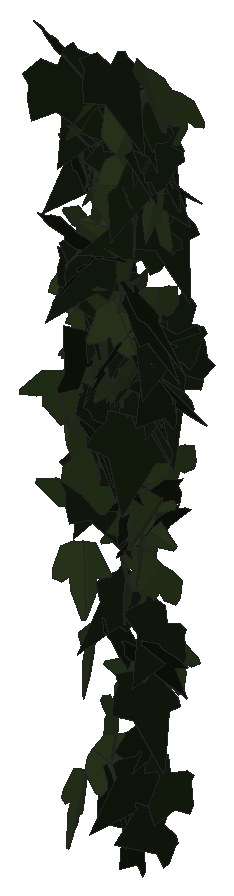
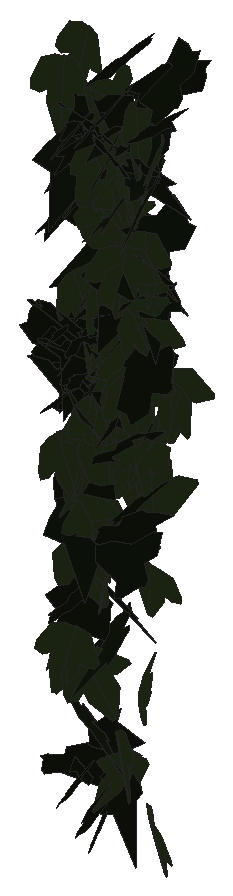
# SketchUp Ruby script. Lengths in inches.
U = 1.inch
M = Sketchup.active_model
def pt(a) = Geom::Point3d.new(a.map { |v| v * U })
def face(e, loops, mat)
  f = e.add_face(loops[0].map { |a| pt(a) })
  loops[1..].each { |l| e.add_face(l.map { |a| pt(a) }).erase! }
  f.material = f.back_material = mat if mat
  f
end
# faces: each face lists its corners as indices into pts; further lists are holes
def faces(e, pts, list, mat = nil) = list.each { |f| face(e, (f[0].is_a?(Array) ? f : [f]).map { |l| l.map { |i| pts[i] } }, mat) }
# xy, xz, yz: faces in a plane at the given z, y or x. An outline is a flat list of corners, or four numbers for a rectangle; further outlines are holes
def ring(l) = l.size == 4 ? [[l[0], l[1]], [l[2], l[1]], [l[2], l[3]], [l[0], l[3]]] : l.each_slice(2).to_a
def flat(e, list, mat, &to3) = list.each { |f| face(e, (f[0].is_a?(Array) ? f : [f]).map { |l| ring(l).map { |u, v| to3.(u, v) } }, mat) }
def xy(e, z, list, mat = nil) = flat(e, list, mat) { |x, y| [x, y, z] }
def xz(e, y, list, mat = nil) = flat(e, list, mat) { |x, z| [x, y, z] }
def yz(e, x, list, mat = nil) = flat(e, list, mat) { |y, z| [x, y, z] }
def lines(e, pts, list) = list.each { |a, b| e.add_line(pt(pts[a]), pt(pts[b])) }
# prism: a flat outline (further loops are holes) pulled along v
def prism(e, loops, v, mat = nil)
  f = face(e, loops, mat); d = Geom::Vector3d.new(v.map { |x| x * U })
  f.pushpull(f.normal.samedirection?(d) ? d.length : -d.length)
end
def box(e, o, s, mat = nil) = prism(e, [[o, [o[0] + s[0], o[1], o[2]], [o[0] + s[0], o[1] + s[1], o[2]], [o[0], o[1] + s[1], o[2]]]], [0, 0, s[2]], mat)
def at(x, y, z, deg = 0) = Geom::Transformation.translation(pt([x, y, z])) * Geom::Transformation.rotation(ORIGIN, Z_AXIS, deg.degrees)
def axes(o, x, y, z) = Geom::Transformation.new([*x, 0, *y, 0, *z, 0, *pt(o).to_a, 1])
def part(name) = M.definitions.add(name)
# library, detail: a bought-in or finely detailed component or shape, given as its bounding box
def library(name, o, s) = part(name).tap { |d| box(d.entities, o, s) }
def detail(e, o, s) = box(e.add_group.entities, o, s)
def put(e, d, t, mat = nil) = e.add_instance(d, t).tap { |i| i.material = mat if mat }
def group(e, t, mat = nil) = e.add_group.tap { |g| g.transformation = t; g.material = mat if mat }.entities
root = M.entities
M.materials.add("efeu1").color = [18, 25, 13]
M.materials.add("efeu2").color = [43, 57, 29]
c1 = part("ivyleaf_10")
p = [[0,0.5,-0.03],[-0.0625,2.02,-0.43],[-0.19,2.01,-0.46],[-0.54,1.05,-0.29],[-0.52,0.625,-0.18],[-0.83,0.76,-0.28],
  [-1.16,0.64,-0.33],[-1.15,0.33,-0.24],[-0.77,-0.39,0.02],[-0.3,-0.51,0.16],[0.04,-0.48,0.23],[-0.02,2.01,-0.4375],
  [-0.06,2.01,-0.43],[0.04,-0.49,0.23],[0.67,-0.49,0.14],[1.38,0.36,-0.2],[1.375,0.51,-0.24],[0.81,0.65,-0.19],
  [0.62,0.59,-0.15],[0.6,1.09,-0.28],[0.5,1.23,-0.31]]
faces(c1.entities,p,[[0,1,2,3,4,5,6,7,8,9,10],[11,12,0,13,14,15,16,17,18,19,20]],"efeu2")
c2 = part("ivyleaf_9")
p = [[1.54,2.16,1.25],[1.36,2.04,1.19],[-0.21,0.99,0.68],[-0.71,1.11,0.82],[-0.85,0.86,0.67],[-0.8,0.17,0.21],
  [-0.9,-0.01,0.1],[-0.67,-0.16,-0.02],[-0.08,-0.08,-0.05],[-0.03,-0.6,-0.4],[0.65,-0.88,-0.66],[0.83,-0.6,-0.49],
  [1.29,-0.42,-0.43],[1.8125,-0.07,-0.26],[1.21,0.44,0.15]]
faces(c2.entities,p,[[0,1,2,3,4,5,6,7,8,9,10,11,12,13,14]],"efeu1")
put(root,c1,axes([551.82,132.52,225.93],[0.90272,0.27085,-0.02157],[-0.0193,-0.01073,-0.94246],[-0.27102,0.90291,-0.00473]))
put(root,c1,axes([551.79,132.23,207.72],[0.74606,-0.58457,0.23749],[0.18704,-0.14635,-0.9478],[0.60261,0.76915,0.00016]))
put(root,c1,axes([551.89,131.1,222.64],[-0.84438,0.29558,-0.21811],[0.19346,-0.10696,-0.8939],[-0.31227,-0.86551,0.03597]))
put(root,c1,axes([552.12,130.91,223.07],[-0.61057,-0.69177,-0.01816],[0.01288,0.01285,-0.92268],[0.69189,-0.6107,0.00115]))
put(root,c2,axes([551.3,131.7,234.54],[0.67517,-0.64526,0.39472],[0.33513,-0.21915,-0.93149],[0.67812,0.75075,0.06735]))
put(root,c1,axes([552.12,132.82,226.29],[-0.06301,-0.82511,0.44369],[0.0616,-0.44737,-0.82322],[0.93481,-0.02613,0.08415]))
put(root,c2,axes([551.42,132.96,224.04],[0.98155,-0.02971,-0.34505],[0.34599,0.12956,0.97308],[0.01517,-1.03233,0.13205]))
put(root,c2,axes([552.12,131.72,231.09],[0.5706,-0.13273,-0.74714],[-0.6309,0.43646,-0.55937],[0.42166,0.83266,0.17411]))
put(root,c1,axes([552.34,132.76,223.61],[-0.46458,-0.79522,0.11666],[-0.01288,-0.12737,-0.91947],[0.80363,-0.46176,0.0527]))
put(root,c2,axes([552.27,133.3125,219],[-0.52467,-0.73699,0.09525],[-0.02342,-0.10014,-0.90384],[0.74275,-0.52376,0.03878]))
put(root,c2,axes([552.59,131.42,226.9375],[-0.1355,0.93298,0.12548],[-0.00562,0.12597,-0.94269],[-0.94137,-0.13505,-0.01243]))
put(root,c1,axes([552.57,131.87,228.29],[-0.89062,0.05393,0.30576],[-0.30524,0.01773,-0.89226],[-0.05676,-0.94148,0.00072]))
put(root,c1,axes([552.375,132.62,223.84],[-0.57631,-0.75007,0.02522],[0.07123,-0.08632,-0.93961],[0.74711,-0.57037,0.10903]))
put(root,c2,axes([551.84,132.36,226.375],[0.32161,-0.89231,0.10139],[0.05079,-0.08945,-0.94834],[0.89662,0.32513,0.01736]))
put(root,c1,axes([552.25,131.57,231.69],[-0.48634,0.81522,0.00802],[0.00541,0.01257,-0.9492],[-0.81524,-0.48624,-0.01108]))
put(root,c1,axes([552.01,132.53,212.6875],[0.10473,-0.36689,0.82699],[0.58913,-0.60416,-0.34264],[0.68662,0.57434,0.16785]))
put(root,c1,axes([552.18,132.22,221.23],[0.4325,0.71572,0.44173],[0.21496,0.38615,-0.83613],[-0.81313,0.48277,0.01391]))
put(root,c1,axes([552.6,131.35,221.3],[0.09304,0.56348,0.72436],[-0.29807,0.70716,-0.51182],[-0.86797,-0.18244,0.2534]))
put(root,c2,axes([552.4,132.27,232.56],[-0.36839,-0.80212,0.38113],[-0.00085,-0.41231,-0.86855],[0.88807,-0.33313,0.15728]))
put(root,c2,axes([552.15,130.82,234.28],[0.13921,-0.73438,-0.69502],[-0.01521,0.69998,-0.74267],[1.01101,0.11165,0.08453]))
put(root,c2,axes([552.93,131.98,231.07],[-0.93048,-0.15791,0.00198],[-0.00094,-0.00629,-0.94377],[0.15792,-0.93046,0.00604]))
put(root,c1,axes([552.6875,132.625,224.95],[-0.48953,-0.7833,0.20194],[0.01391,-0.24416,-0.91333],[0.80879,-0.4699,0.13794]))
put(root,c1,axes([552.75,132.4,227.34],[-0.50526,-0.80101,-0.05026],[0.06353,0.01929,-0.94606],[0.80007,-0.50739,0.04338]))
put(root,c1,axes([552.37,131.6,216.45],[0.91454,-0.01963,0.28681],[0.28667,-0.00966,-0.91474],[0.02162,0.95841,-0.00335]))
put(root,c2,axes([552.6,133.16,221.54],[-0.36059,-0.83056,0.17307],[0.00773,-0.19126,-0.90176],[0.84836,-0.35128,0.08178]))
put(root,c2,axes([551.95,132.71,217.49],[0.58855,-0.42318,0.60133],[0.52116,-0.30329,-0.72352],[0.51872,0.78486,0.04464]))
put(root,c1,axes([552.93,132.49,210.43],[0.54202,-0.50406,-0.50402],[-0.25961,0.45011,-0.72932],[0.66387,0.58756,0.12631]))
put(root,c1,axes([552.75,131.14,218.91],[-0.94233,-0.44249,0.09803],[0.0915,0.03576,1.04103],[-0.44389,0.94674,0.0065]))
put(root,c1,axes([552.87,131.72,232.84],[0.02812,-0.9489,-0.20865],[0.01447,0.20912,-0.9491],[0.97146,0.02435,0.02018]))
put(root,c2,axes([553.125,131.6875,227.49],[-0.94346,-0.08712,-0.10658],[0.1105,-0.0391,-0.94621],[0.08208,-0.94865,0.04879]))
put(root,c2,axes([552.71,131.4,223.55],[0.22376,0.39828,0.90514],[-0.43122,-0.79584,0.45679],[0.88992,-0.48577,-0.00625]))
put(root,c1,axes([552.9375,132.49,227.91],[-0.82883,-0.45028,-0.04002],[0.02278,0.04187,-0.94289],[0.45148,-0.82874,-0.0259]))
put(root,c1,axes([553.1,131.43,231.53],[0.40048,-0.74693,-0.47849],[-0.18157,0.44485,-0.84639],[0.86827,0.43754,0.0437]))
put(root,c2,axes([552.12,131.23,228.09],[0.3936,-0.47353,0.75117],[0.72203,-0.3076,-0.57223],[0.51687,0.79029,0.22736]))
put(root,c2,axes([552.875,132.71,226.125],[-0.40295,-0.85604,0.03989],[-0.01238,-0.03825,-0.94612],[0.85688,-0.40311,0.00509]))
put(root,c2,axes([552.97,131.92,227.14],[0.42175,0.82441,0.1255],[0.06955,0.10537,-0.92592],[-0.831,0.42722,-0.0138]))
put(root,c1,axes([552.73,132.09,220.76],[0.55421,-0.62262,0.39865],[0.35933,-0.20857,-0.8253],[0.64611,0.65006,0.11703]))
put(root,c2,axes([552.32,131.66,231.4],[0.73739,-0.47364,0.36848],[0.34811,-0.13789,-0.87387],[0.4888,0.81272,0.06648]))
put(root,c2,axes([552.625,131.71,219.15],[0.36461,-0.78084,-0.35188],[0.02451,0.39179,-0.84402],[0.85612,0.32133,0.17402]))
put(root,c2,axes([552.97,131.93,222.57],[0.53336,-0.38539,-0.68611],[-0.37603,0.60329,-0.63118],[0.69129,0.62551,0.18603]))
put(root,c1,axes([553.48,131.23,225.12],[-0.61871,0.66022,0.22592],[-0.38153,-0.06725,-0.84832],[-0.58427,-0.65522,0.31471]))
put(root,c1,axes([553.07,131.87,209.37],[0.12068,0.64943,0.6144],[0.12094,0.60241,-0.66052],[-0.88579,0.17073,-0.00647]))
put(root,c1,axes([553.15,132.99,220.67],[-0.00013,-1.00563,-0.30699],[0.0436,-0.30673,1.00477],[-1.05054,-0.0126,0.04174]))
put(root,c1,axes([553.43,131.57,230.79],[0.23592,-0.93089,-0.15971],[-0.05693,0.1503,-0.96015],[0.94277,0.24202,-0.01802]))
put(root,c2,axes([553.75,131.6,208.56],[0.39458,0.07969,-0.90298],[-0.8919,-0.14185,-0.40226],[-0.16198,0.97517,0.01528]))
put(root,c2,axes([552.82,132.01,220.91],[0.31076,-0.74062,0.5461],[0.20329,-0.5069,-0.80314],[0.89745,0.37128,-0.00717]))
put(root,c2,axes([553.06,132.2,224.99],[0.4874,-0.71309,-0.3513],[-0.14841,0.3232,-0.86196],[0.78095,0.50647,0.05544]))
put(root,c1,axes([553.85,132.35,230.78],[-0.48217,-0.75284,0.31794],[-0.1775,-0.26387,-0.89399],[0.79772,-0.51376,-0.00674]))
put(root,c2,axes([553.87,131.99,215.51],[-0.8486,0.08778,-0.20637],[0.1971,-0.09341,-0.8502],[-0.10699,-0.86832,0.0706]))
put(root,c2,axes([553.16,131.86,222],[0.21998,-0.89706,0.27124],[0.07375,-0.26118,-0.9236],[0.93426,0.23184,0.00904]))
put(root,c1,axes([553.67,132.875,222.48],[-0.4573,-0.8071,0.09596],[0.07205,-0.14992,-0.91764],[0.80958,-0.44256,0.13587]))
put(root,c1,axes([553.57,131.13,230.21],[-0.01665,-0.10873,-1.00511],[0.17915,0.98902,-0.10996],[0.99497,-0.1799,0.00297]))
put(root,c2,axes([553.18,132.02,230.07],[0.61843,-0.72069,-0.18351],[-0.09655,0.15884,-0.94919],[0.73739,0.62522,0.02962]))
put(root,c2,axes([553.37,131.99,214.21],[0.77695,-0.3726,-0.43778],[-0.32469,0.32297,-0.85112],[0.47441,0.83126,0.13445]))
put(root,c1,axes([553.77,132.52,226.23],[0.08921,-0.94739,-0.00917],[-0.00355,0.00888,-0.95157],[0.94742,0.08924,-0.0027]))
put(root,c2,axes([553.51,132.3,225.83],[-0.17337,-0.91347,0.07339],[-0.00791,-0.0732,-0.92976],[0.91638,-0.17345,0.00586]))
put(root,c1,axes([554.07,131.47,226.875],[-0.01533,-0.01827,-1.01117],[-0.24305,0.98171,-0.01405],[0.98169,0.24276,-0.01927]))
put(root,c1,axes([553.74,131.875,223.65],[-0.21767,-0.75169,-0.50229],[0.21487,0.45882,-0.77975],[0.87816,-0.29859,0.06629]))
put(root,c2,axes([553.73,132.86,223.78],[-0.4012,-0.8429,0.05079],[0.01598,-0.0638,-0.93258],[0.84428,-0.39934,0.04179]))
put(root,c1,axes([553.9375,132.5,221.79],[-0.76243,-0.48851,-0.03012],[0.02255,0.02065,-0.90549],[0.48892,-0.76275,-0.00522]))
put(root,c1,axes([553.99,131.39,226.33],[-0.87886,-0.3293,0.02358],[-0.02201,-0.00846,-0.93853],[0.32941,-0.87914,0.0002]))
put(root,c2,axes([554.2,132.0625,231.52],[-0.9102,0.1357,-0.27704],[0.27859,-0.00914,-0.91974],[-0.1325,-0.95138,-0.03068]))
put(root,c1,axes([554.33,132.08,228.59],[0.14684,0.32298,0.89101],[-0.4303,-0.78063,0.35388],[0.84443,-0.45396,0.02539]))
put(root,c1,axes([554.37,132.41,212.68],[-0.57959,-0.55475,0.46155],[-0.33939,-0.31289,-0.80226],[0.63686,-0.6716,-0.00749]))
put(root,c2,axes([553.99,132.86,207.57],[-0.22977,-0.33,0.7627],[-0.20548,-0.74418,-0.38389],[0.80522,-0.28407,0.11967]))
put(root,c2,axes([554.55,132.625,222.48],[-0.70506,0.5943,0.03616],[-0.02468,0.02683,-0.92211],[-0.59489,-0.70548,-0.0046]))
put(root,c2,axes([553.93,132.55,224.97],[-0.34234,-0.88233,0.07973],[0.01363,-0.09071,-0.94532],[0.88582,-0.33959,0.04535]))
put(root,c1,axes([554.03,131.23,224.17],[-0.28259,0.92203,0.14813],[-0.04196,0.14207,-0.96436],[-0.93291,-0.28569,-0.0015]))
put(root,c2,axes([554.42,131.07,225.07],[-0.50474,0.75424,-0.39077],[0.22457,-0.31989,-0.90751],[-0.81924,-0.55239,-0.00802]))
put(root,c2,axes([553.85,132.88,223.01],[-0.55557,-0.32246,-0.65463],[0.60861,0.2492,-0.63927],[0.40263,-0.82164,0.06303]))
put(root,c1,axes([554.26,131.45,216.29],[0.4126,-0.49873,-0.61269],[-0.08737,0.65818,-0.59458],[0.78517,0.33532,0.25581]))
put(root,c2,axes([553.74,131.45,234.5625],[0.29479,-0.9262,-0.20577],[0.0568,0.23231,-0.96431],[0.94708,0.27435,0.12188]))
put(root,c1,axes([554.24,132.16,218.21],[-0.52516,-0.74176,-0.23016],[0.15737,0.17044,-0.90838],[0.76054,-0.54746,0.02903]))
put(root,c1,axes([553.72,132.27,218.24],[-0.40256,-0.10954,-0.83439],[0.83997,-0.10885,-0.39097],[-0.05145,-0.92,0.1456]))
put(root,c2,axes([554.95,131.85,210.67],[-0.58106,0.65738,0.34874],[-0.24195,0.25152,-0.87726],[-0.70372,-0.62927,0.01367]))
put(root,c1,axes([554.43,132.13,224.25],[0.30671,-0.88746,-0.15027],[-0.04773,0.14249,-0.93896],[0.89882,0.31039,0.00142]))
put(root,c1,axes([554.45,131.55,231.07],[-0.52004,-0.8198,-0.09776],[0.04568,0.08678,-0.9708],[0.82434,-0.52198,-0.00787]))
put(root,c2,axes([554.64,132.25,218.01],[0.01691,0.94048,-0.03148],[-0.0003,-0.03148,-0.94063],[-0.94101,0.01691,-0.00026]))
put(root,c2,axes([554.1,132.19,206.82],[0.031,-0.43481,0.73962],[0.01419,-0.73974,-0.43548],[0.85785,0.02795,-0.01952]))
put(root,c2,axes([554.0625,131.82,231.05],[0.69096,-0.54814,-0.36589],[-0.2669,0.25197,-0.88149],[0.60258,0.74014,0.02911]))
put(root,c1,axes([554.46,131.46,224.16],[0.13886,-0.89862,-0.26963],[0.02743,0.27634,-0.90685],[0.9378,0.12497,0.06645]))
put(root,c2,axes([553.91,132.45,223.46],[0.49198,-0.77447,0.10572],[0.07515,-0.07748,-0.91727],[0.77804,0.49721,0.02174]))
put(root,c2,axes([554.28,131.9,232.97],[-0.56445,-0.70278,-0.37824],[0.2831,0.25685,-0.8997],[0.74621,-0.62905,0.05521]))
put(root,c2,axes([554.02,131.83,232.67],[0.39717,-0.89256,-0.12893],[-0.00528,0.13858,-0.9756],[0.90181,0.39391,0.05107]))
put(root,c1,axes([554.97,132.19,216.55],[-0.72266,-0.23715,0.5618],[-0.5048,-0.25608,-0.75744],[0.34211,-0.8788,0.06911]))
put(root,c1,axes([554.25,131.17,226.13],[-0.33244,-0.84368,-0.23717],[0.47786,0.03813,-0.80546],[0.73464,-0.40659,0.4166]))
put(root,c1,axes([554.52,130.91,232.5625],[0.11554,0.59728,-0.82362],[0.13343,0.81285,0.6082],[1.00861,-0.17596,0.01389]))
put(root,c2,axes([554.51,131.89,224.41],[0.59241,0.75239,-0.08961],[-0.04618,-0.07768,-0.95755],[-0.7563,0.59409,-0.01172]))
put(root,c1,axes([554.41,131.78,229.97],[0.59013,-0.67433,0.32163],[0.33077,-0.13169,-0.88299],[0.66989,0.65906,0.15265]))
put(root,c2,axes([555.26,132.09,229.07],[-0.6965,-0.26249,0.58932],[-0.55709,-0.19263,-0.74421],[0.32533,-0.8918,-0.01271]))
put(root,c1,axes([554.84,132.28,226.33],[-0.27859,-0.86412,0.23379],[-0.00259,-0.24407,-0.90521],[0.89519,-0.26962,0.07014]))
put(root,c1,axes([554.44,130.49,231.125],[-0.06348,-0.33137,-0.92792],[0.56107,0.75222,-0.30701],[0.80997,-0.54703,0.13994]))
put(root,c1,axes([554.66,131.875,219.71],[0.21574,-0.63239,-0.65166],[0.24601,0.68545,-0.58374],[0.8741,-0.03683,0.32512]))
put(root,c2,axes([555.08,131.65,219.72],[-0.05461,0.72871,-0.52813],[0.00366,-0.52891,-0.73018],[-0.89996,-0.04637,0.02908]))
put(root,c1,axes([554.83,131.75,219.55],[0.2416,0.82501,-0.27116],[-0.18361,-0.22657,-0.85293],[-0.84879,0.28384,0.10732]))
put(root,c1,axes([554.91,131.87,229.6],[0.92001,-0.16495,-0.2351],[-0.19973,0.19943,-0.92154],[0.20636,0.9284,0.15618]))
put(root,c2,axes([554.87,131.51,231.8],[-0.58532,-0.77968,-0.08939],[0.04252,0.07984,-0.97484],[0.78364,-0.5867,-0.01387]))
put(root,c1,axes([554.88,132.68,213.64],[-0.88705,-0.12652,-0.11291],[0.11225,0.01265,-0.89602],[0.1271,-0.89412,0.0033]))
put(root,c2,axes([554.86,131.56,209.46],[0.02648,-0.14233,-0.90205],[0.39527,-0.81173,0.13968],[-0.82323,-0.39432,0.03805]))
put(root,c2,axes([554.51,131.79,231.53],[0.30678,-0.66818,-0.61278],[-0.01755,0.64241,-0.70928],[0.90645,0.23858,0.19365]))
put(root,c2,axes([555.53,131.98,232.16],[-0.95354,0.13908,0.1557],[-0.16823,-0.08078,-0.95813],[-0.12363,-0.96279,0.10288]))
put(root,c2,axes([554.85,131.32,221.92],[-0.49608,-0.72428,-0.23086],[0.17453,0.15979,-0.87635],[0.73988,-0.52332,0.05193]))
put(root,c2,axes([554.55,132.625,222.84],[0.0937,-0.92083,-0.09485],[0.15619,0.10969,-0.91064],[0.91243,0.07579,0.16563]))
put(root,c1,axes([555.15,132.73,220.57],[-0.34963,-0.80997,0.20365],[-0.05804,-0.19668,-0.88188],[0.83316,-0.3536,0.02403]))
put(root,c2,axes([554.77,132.6,225.1875],[-0.14353,-0.88987,0.27389],[0.02492,-0.2807,-0.89892],[0.93073,-0.12972,0.0663]))
put(root,c2,axes([555.05,131.875,231.04],[0.78323,0.42115,-0.40357],[-0.48625,0.09824,-0.84118],[-0.32217,0.87559,0.28849]))
put(root,c1,axes([555.19,131.05,218.08],[0.49491,-0.6377,-0.44423],[-0.13069,0.45086,-0.79283],[0.7661,0.48887,0.15172]))
put(root,c2,axes([555.18,132.4375,209.23],[-0.65023,-0.62372,0.01385],[-0.00554,-0.01423,-0.90099],[0.62385,-0.65022,0.00643]))
put(root,c1,axes([555.01,132.28,219.24],[0.1507,-0.54383,0.75517],[0.18291,-0.73277,-0.5642],[0.91246,0.23671,-0.01162]))
put(root,c2,axes([555.09,132.76,224.15],[-0.72476,-0.51666,-0.29892],[0.26061,0.14912,-0.88962],[0.53701,-0.76967,0.0283]))
put(root,c2,axes([554.63,132.43,232.32],[0.39615,-0.86843,0.04033],[0.0386,-0.0267,-0.95422],[0.86851,0.39731,0.02401]))
put(root,c2,axes([555.75,132.51,223.91],[0.08694,0.0547,0.94184],[-0.85337,0.40785,0.05508],[-0.40226,-0.85339,0.08669]))
put(root,c2,axes([554.84,131.33,226.47],[0.71042,-0.60476,-0.29924],[-0.23473,0.18587,-0.93292],[0.6326,0.74813,-0.01012]))
put(root,c1,axes([555.27,131.53,234.7],[-0.91081,0.30113,-0.00657],[-0.00155,-0.02561,-0.95898],[-0.3012,-0.91048,0.0248]))
put(root,c2,axes([555.64,132.88,225.38],[-0.92898,0.01646,-0.0363],[0.03624,-0.00378,-0.92912],[-0.0166,-0.92968,0.00313]))
put(root,c2,axes([554.49,132.42,223.28],[0.55695,-0.43869,0.65103],[0.52388,-0.38681,-0.70882],[0.58468,0.76448,0.01495]))
put(root,c2,axes([555.25,132.22,214.74],[-0.24045,-0.75901,0.39154],[-0.05803,-0.39131,-0.79419],[0.85208,-0.24084,0.0564]))
put(root,c1,axes([555.59,132.25,233.79],[-0.942,0.03054,0.18132],[-0.18146,-0.00156,-0.94247],[-0.02969,-0.95929,0.00731]))
put(root,c2,axes([555,131.53,212.72],[0.17325,-0.91476,-0.16218],[0.00143,0.16524,-0.93048],[0.92903,0.17034,0.03168]))
put(root,c2,axes([555.4,131.9,207.76],[-0.32311,-0.36797,0.79211],[-0.1585,-0.80585,-0.43901],[0.8589,-0.28714,0.21697]))
put(root,c2,axes([555.2,131.22,214.27],[0.82556,0.26468,-0.13252],[-0.12453,-0.04563,-0.86693],[-0.26853,0.83488,-0.00537]))
put(root,c2,axes([555.08,132.36,229.3],[0.27908,-0.90035,-0.1745],[-0.00192,0.18183,-0.94122],[0.9171,0.27436,0.05113]))
put(root,c1,axes([555.45,131.46,230.77],[0.77379,-0.54789,0.07739],[0.06602,-0.04067,-0.94811],[0.54938,0.77659,0.00494]))
put(root,c2,axes([554.96,131.19,226.92],[0.72357,-0.65778,0.07693],[0.064,-0.04395,-0.97781],[0.65916,0.72632,0.0105]))
put(root,c2,axes([555.32,131.97,223.54],[-0.0894,-0.58409,0.72232],[-0.01094,-0.72494,-0.58756],[0.92886,-0.06476,0.0626]))
